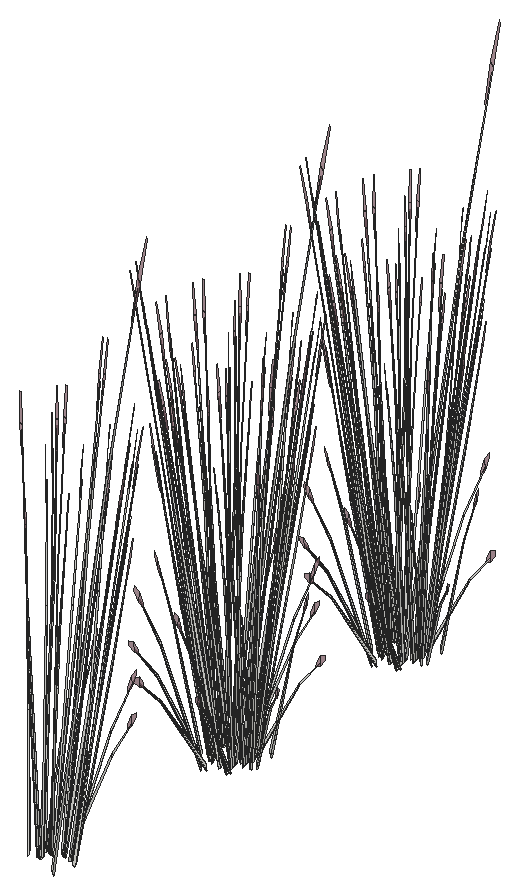
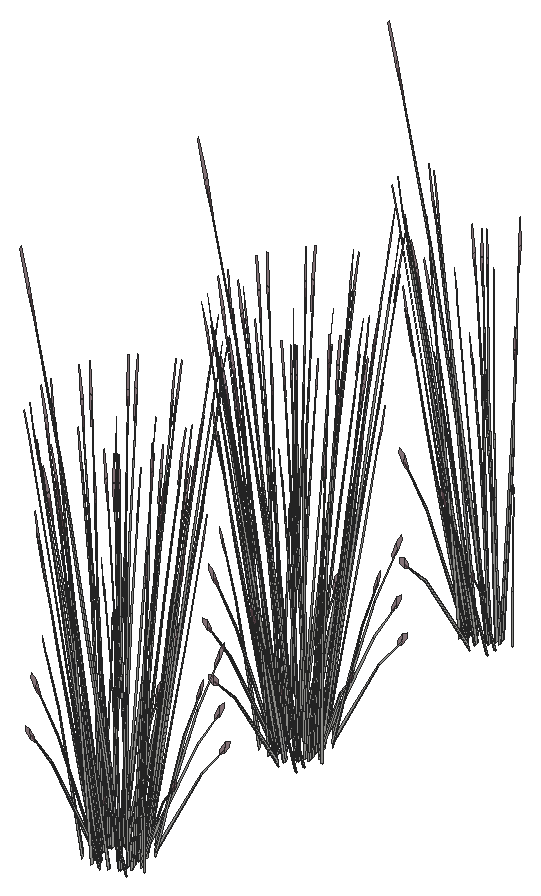
# SketchUp Ruby script. Lengths in inches.
U = 1.inch
M = Sketchup.active_model
def pt(a) = Geom::Point3d.new(a.map { |v| v * U })
def face(e, loops, mat)
  f = e.add_face(loops[0].map { |a| pt(a) })
  loops[1..].each { |l| e.add_face(l.map { |a| pt(a) }).erase! }
  f.material = f.back_material = mat if mat
  f
end
# faces: each face lists its corners as indices into pts; further lists are holes
def faces(e, pts, list, mat = nil) = list.each { |f| face(e, (f[0].is_a?(Array) ? f : [f]).map { |l| l.map { |i| pts[i] } }, mat) }
# xy, xz, yz: faces in a plane at the given z, y or x. An outline is a flat list of corners, or four numbers for a rectangle; further outlines are holes
def ring(l) = l.size == 4 ? [[l[0], l[1]], [l[2], l[1]], [l[2], l[3]], [l[0], l[3]]] : l.each_slice(2).to_a
def flat(e, list, mat, &to3) = list.each { |f| face(e, (f[0].is_a?(Array) ? f : [f]).map { |l| ring(l).map { |u, v| to3.(u, v) } }, mat) }
def xy(e, z, list, mat = nil) = flat(e, list, mat) { |x, y| [x, y, z] }
def xz(e, y, list, mat = nil) = flat(e, list, mat) { |x, z| [x, y, z] }
def yz(e, x, list, mat = nil) = flat(e, list, mat) { |y, z| [x, y, z] }
def lines(e, pts, list) = list.each { |a, b| e.add_line(pt(pts[a]), pt(pts[b])) }
# prism: a flat outline (further loops are holes) pulled along v
def prism(e, loops, v, mat = nil)
  f = face(e, loops, mat); d = Geom::Vector3d.new(v.map { |x| x * U })
  f.pushpull(f.normal.samedirection?(d) ? d.length : -d.length)
end
def box(e, o, s, mat = nil) = prism(e, [[o, [o[0] + s[0], o[1], o[2]], [o[0] + s[0], o[1] + s[1], o[2]], [o[0], o[1] + s[1], o[2]]]], [0, 0, s[2]], mat)
def at(x, y, z, deg = 0) = Geom::Transformation.translation(pt([x, y, z])) * Geom::Transformation.rotation(ORIGIN, Z_AXIS, deg.degrees)
def axes(o, x, y, z) = Geom::Transformation.new([*x, 0, *y, 0, *z, 0, *pt(o).to_a, 1])
def part(name) = M.definitions.add(name)
# library, detail: a bought-in or finely detailed component or shape, given as its bounding box
def library(name, o, s) = part(name).tap { |d| box(d.entities, o, s) }
def detail(e, o, s) = box(e.add_group.entities, o, s)
def put(e, d, t, mat = nil) = e.add_instance(d, t).tap { |i| i.material = mat if mat }
def group(e, t, mat = nil) = e.add_group.tap { |g| g.transformation = t; g.material = mat if mat }.entities
root = M.entities
M.materials.add("LightPink_Translucent").color = [144, 107, 117]
M.materials["LightPink_Translucent"].alpha = 0.75
c1 = part("blade")
p = [[2.15,0.21,22],[0,0.17,0],[0.09,0.45,0],[2.18,0.31,22],[2.29,0.31,22],[0.38,0.45,0],
  [2.48,0.24,33],[2.49,0.24,33],[2.48,0.22,33]]
faces(c1.entities,p,[[0,1,2,3],[4,5,2,3],[6,3,4,7],[8,0,3,6]])
c2 = part("seeds")
p = [[0.3,-0.1,1.38],[-0.01,-0.03,1.59],[-0.01,-0.03,0.03],[0.14,-0.07,-0.07],[0.29,-0.03,3],[0.15,0.01,3.11]]
faces(c2.entities,p,[[0,1,2,3],[1,0,4,5]],"LightPink_Translucent")
c3 = part("blade with seeds")
put(c3.entities,c1,at(0,0,0))
put(c3.entities,c2,axes([2.4,0.25,30.99],[1.5799,-0.05474,1.17369],[-0.12525,1.92788,0.29478],[-0.07173,-0.02425,1.56792]))
put(root,c3,axes([400.47,80.36,4.73],[-0.08753,-0.42921,0.48003],[0.34336,-0.07449,0.3958],[-0.1012,0.10094,0.9933]))
put(root,c3,axes([400.41,80.28,4.73],[-0.2423,-0.19613,0.0643],[0.14107,-0.2793,0.50621],[-0.07768,0.0903,0.77189]))
put(root,c3,axes([400.6875,80.22,5.05],[0.30722,-0.06665,0.35414],[0.08112,0.381,-0.4572],[-0.08804,0.10234,0.87481]))
put(root,c3,axes([399.5,80.05,4.71],[0.04504,0.01251,1.77383],[0.13934,0.41205,-0.16761],[-0.0922,0.10815,0.31391]))
put(root,c3,axes([403.32,81.08,4.73],[-0.01777,0.35463,0.0643],[-0.26836,-0.00972,0.50621],[0.1028,0.03711,0.77189]))
put(root,c3,axes([403.34,80.97,4.73],[-0.26024,0.30729,0.48003],[-0.22444,-0.32634,0.3958],[0.1221,0.05668,0.9933]))
put(root,c3,axes([399.99,81.3,5.65],[0.31145,0.12449,-0.06488],[-0.0958,0.38314,-0.29416],[-0.05094,0.05817,0.97024]))
put(root,c3,axes([402.52,81.32,5.05],[-0.05451,-0.37564,0.35414],[0.31161,-0.09919,-0.4572],[0.0837,0.10765,0.87481]))
put(root,c3,axes([402.72,79.16,4.47],[-0.30498,-0.24231,1.38283],[0.32203,-0.37727,0.59665],[0.0984,0.22736,1.33663]))
put(root,c3,axes([400.53,80.18,5.03],[0.32648,0.25715,-0.1216],[-0.18809,0.3724,-0.67495],[-0.09224,0.12945,1.02557]))
put(root,c3,axes([402.49,81.52,5.03],[0.21031,-0.39918,-0.1216],[0.30457,0.22997,-0.67495],[0.10587,0.11278,1.02557]))
put(root,c3,axes([401.1,80.98,5.05],[0.23881,-0.24554,0.35414],[0.22606,0.28036,-0.4572],[-0.0344,0.14245,0.87481]))
put(root,c3,axes([402.21,81.85,4.71],[0.00104,-0.05646,1.77383],[0.30246,-0.2491,-0.16761],[0.10506,0.08891,0.31391]))
put(root,c3,axes([400.88,81.2,4.73],[-0.29004,-0.02173,0.0643],[0.00795,-0.32812,0.50621],[-0.03035,0.12569,0.77189]))
put(root,c3,axes([400.98,81.23,4.73],[-0.25132,-0.3182,0.48003],[0.2669,-0.27442,0.3958],[-0.04636,0.14929,0.9933]))
put(root,c3,axes([401.77,81.38,5.05],[0.1064,-0.35863,0.35414],[0.31043,0.1046,-0.4572],[0.02846,0.14439,0.87481]))
put(root,c3,axes([402.56,81.66,4.73],[-0.16041,0.29625,0.0643],[-0.22843,-0.17248,0.50621],[0.07385,0.09498,0.77189]))
put(root,c3,axes([402.1875,82.66,5.65],[0.2439,-0.26754,-0.06488],[0.22348,0.29302,-0.29416],[0.01573,0.08303,0.97024]))
put(root,c3,axes([402.63,81.58,4.73],[-0.35104,0.10702,0.48003],[-0.06092,-0.41983,0.3958],[0.08256,0.12373,0.9933]))
put(root,c3,axes([401.67,81.71,4.73],[-0.26007,0.1585,0.0643],[-0.12729,-0.28902,0.50621],[0.02512,0.1274,0.77189]))
put(root,c3,axes([400.15,81.25,4.72],[-0.00877,0.09229,1.74944],[0.24897,0.32105,-0.27667],[-0.06518,0.15182,0.14031]))
put(root,c3,axes([400.95,81.05,5.4],[0.3879,0.02311,-0.13498],[-0.0106,0.43749,-0.74919],[-0.02694,0.1685,1.13838]))
put(root,c3,axes([401.67,81.53,5.03],[0.34538,-0.21713,-0.1216],[0.16972,0.38536,-0.67495],[0.04557,0.16239,1.02557]))
put(root,c3,axes([401.77,81.68,5.0625],[-0.34777,-0.12192,0.53283],[0.11892,-0.40083,0.43934],[0.0209,0.15763,1.10256]))
put(root,c3,axes([400.125,82.2,4.71],[0.04004,-0.02816,1.77383],[0.33095,0.18728,-0.16761],[-0.00778,0.15594,0.31391]))
put(root,c3,axes([401.58,82.4,4.72],[0.04474,0.0751,1.74944],[0.36104,0.0295,-0.27667],[0.03631,0.16562,0.14031]))
put(root,c3,axes([401.89,98.37,4.72],[-0.05398,-0.06539,1.74944],[-0.36026,0.04145,-0.27667],[-0.0575,-0.15639,0.14031]))
put(root,c3,axes([403.51,99.17,4.72],[-0.00341,-0.09282,1.74944],[-0.28775,-0.26825,-0.27667],[0.04449,-0.16261,0.14031]))
put(root,c3,axes([403.43,98.83,4.71],[-0.03584,0.03562,1.77383],[-0.35118,-0.12018,-0.16761],[-0.01271,-0.15545,0.31391]))
put(root,c3,axes([401.52,98.15,4.71],[-0.00658,0.0559,1.77383],[-0.32474,0.20287,-0.16761],[-0.09556,-0.1037,0.31391]))
put(root,c3,axes([401.45,99.14,5.09],[0.39316,-0.11987,0.53763],[0.06823,0.47021,0.4433],[-0.09247,-0.13858,1.11249]))
put(root,c3,axes([402.34,99.23,4.73],[0.34777,0.12192,0.48003],[-0.11892,0.40083,0.3958],[-0.0209,-0.15763,0.9933]))
put(root,c3,axes([402.4375,99.375,5.03],[-0.34538,0.21713,-0.1216],[-0.16972,-0.38536,-0.67495],[-0.04557,-0.16239,1.02557]))
put(root,c3,axes([403.15,99.86,5.03],[-0.3879,-0.02311,-0.1216],[0.0106,-0.43749,-0.67495],[0.02694,-0.1685,1.02557]))
put(root,c3,axes([402.43,99.2,4.73],[0.26007,-0.1585,0.0643],[0.12729,0.28902,0.50621],[-0.02512,-0.1274,0.77189]))
put(root,c3,axes([401.54,99.25,4.73],[0.16041,-0.29625,0.0643],[0.22843,0.17248,0.50621],[-0.07385,-0.09498,0.77189]))
put(root,c3,axes([402.33,99.53,5.05],[-0.1064,0.35863,0.35414],[-0.31043,-0.1046,-0.4572],[-0.02846,-0.14439,0.87481]))
put(root,c3,axes([403.125,99.68,4.73],[0.25132,0.3182,0.48003],[-0.2669,0.27442,0.3958],[0.04636,-0.14929,0.9933]))
put(root,c3,axes([401.61,99.21,5.43],[-0.23555,0.44708,-0.13619],[-0.34112,-0.25757,-0.75594],[-0.11858,-0.12631,1.14864]))
put(root,c3,axes([403.22,99.71,4.73],[0.29004,0.02173,0.0643],[-0.00795,0.32812,0.50621],[0.03035,-0.12569,0.77189]))
put(root,c3,axes([403,99.93,5.05],[-0.23881,0.24554,0.35414],[-0.22606,-0.28036,-0.4572],[0.0344,-0.14245,0.87481]))
put(root,c3,axes([400.71,99.09,4.72],[-0.07594,-0.00329,1.74944],[-0.24177,0.32918,-0.27667],[-0.129,-0.06726,0.14031]))
put(root,c3,axes([403.58,100.72,5.03],[-0.32648,-0.25715,-0.1216],[0.18809,-0.3724,-0.67495],[0.09224,-0.12945,1.02557]))
put(root,c3,axes([401.59,99.59,5.05],[0.05451,0.37564,0.35414],[-0.31161,0.09919,-0.4572],[-0.0837,-0.10765,0.87481]))
put(root,c3,axes([400.65,99.83,5.09],[0.29147,-0.34417,0.53763],[0.25138,0.3655,0.4433],[-0.13675,-0.06349,1.11249]))
put(root,c3,axes([404.38,100.61,4.71],[-0.0461,-0.00354,1.77383],[-0.19143,-0.37951,-0.16761],[0.07688,-0.12478,0.31391]))
put(root,c3,axes([400.78,99.83,4.73],[0.01777,-0.35463,0.0643],[0.26836,0.00972,0.50621],[-0.1028,-0.03711,0.77189]))
put(root,c3,axes([403.42,100.6875,5.05],[-0.30722,0.06665,0.35414],[-0.08112,-0.381,-0.4572],[0.08804,-0.10234,0.87481]))
put(root,c3,axes([403.7,100.63,4.73],[0.2423,0.19613,0.0643],[-0.14107,0.2793,0.50621],[0.07768,-0.0903,0.77189]))
put(root,c3,axes([403.63,100.55,4.73],[0.08753,0.42921,0.48003],[-0.34336,0.07449,0.3958],[0.1012,-0.10094,0.9933]))
put(root,c3,axes([404.55,101.07,4.72],[0.04898,-0.07104,1.74944],[-0.06269,-0.43574,-0.27667],[0.12289,-0.08262,0.14031]))
put(root,c3,axes([400.42,99.37,4.71],[0.02617,0.04654,1.77383],[-0.12614,0.41836,-0.16761],[-0.12775,0.00303,0.31391]))
put(root,c3,axes([400.97,100.09,5.05],[0.20082,0.29199,0.35414],[-0.2293,0.2764,-0.4572],[-0.1165,-0.04206,0.87481]))
put(root,c3,axes([400.91,99.91,5.03],[-0.0189,0.47427,-0.1216],[-0.35781,-0.01296,-0.67495],[-0.13781,-0.03295,1.02557]))
put(root,c3,axes([403.59,101.73,5.03],[-0.17758,-0.42229,-0.1216],[0.31518,-0.20752,-0.67495],[0.13282,-0.05572,1.02557]))
put(root,c3,axes([403.47,101.6,5.05],[-0.29332,-0.1301,0.35414],[0.08555,-0.37955,-0.4572],[0.11809,-0.0348,0.87481]))
put(root,c3,axes([400.4,100.91,4.73],[0.09971,-0.42522,0.48003],[0.32782,0.1454,0.3958],[-0.12892,0.02555,0.9933]))
put(root,c3,axes([400.37,100.79,4.73],[-0.12963,-0.31798,0.0643],[0.23638,-0.15564,0.50621],[-0.1042,0.03071,0.77189]))
put(root,c3,axes([403.73,101.72,4.73],[0.12963,0.31798,0.0643],[-0.23638,0.15564,0.50621],[0.1042,-0.03071,0.77189]))
put(root,c3,axes([403.71,101.61,4.73],[-0.09971,0.42522,0.48003],[-0.32782,-0.1454,0.3958],[0.12892,-0.02555,0.9933]))
put(root,c3,axes([400.64,100.91,5.05],[0.29332,0.1301,0.35414],[-0.08555,0.37955,-0.4572],[-0.11809,0.0348,0.87481]))
put(root,c3,axes([404.3,102.98,4.71],[-0.03191,-0.04083,1.77383],[0.06981,-0.43764,-0.16761],[0.12571,-0.02796,0.31391]))
put(root,c3,axes([400.14,101.21,4.72],[-0.05763,0.06055,1.74944],[0.0049,0.44239,-0.27667],[-0.13211,0.05753,0.14031]))
put(root,c3,axes([400.51,100.78,5.03],[0.17758,0.42229,-0.1216],[-0.31518,0.20752,-0.67495],[-0.13282,0.05572,1.02557]))
put(root,c3,axes([403.19,102.61,5.03],[0.0189,-0.47427,-0.1216],[0.35781,0.01296,-0.67495],[0.13781,0.03295,1.02557]))
put(root,c3,axes([403.14,102.42,5.05],[-0.20082,-0.29199,0.35414],[0.2293,-0.2764,-0.4572],[0.1165,0.04206,0.87481]))
put(root,c3,axes([403.5,102.32,4.72],[0.07571,-0.00789,1.74944],[0.20767,-0.36231,-0.27667],[0.13467,0.04783,0.14031]))
put(root,c3,axes([400.47,101.97,4.73],[-0.08753,-0.42921,0.48003],[0.34336,-0.07449,0.3958],[-0.1012,0.10094,0.9933]))
put(root,c3,axes([400.41,101.88,4.73],[-0.2423,-0.19613,0.0643],[0.14107,-0.2793,0.50621],[-0.07768,0.0903,0.77189]))
put(root,c3,axes([400.6875,101.82,5.05],[0.30722,-0.06665,0.35414],[0.08112,0.381,-0.4572],[-0.08804,0.10234,0.87481]))
put(root,c3,axes([399.5,101.65,4.71],[0.04504,0.01251,1.77383],[0.13934,0.41205,-0.16761],[-0.0922,0.10815,0.31391]))
put(root,c3,axes([403.32,102.68,4.73],[-0.01777,0.35463,0.0643],[-0.26836,-0.00972,0.50621],[0.1028,0.03711,0.77189]))
put(root,c3,axes([403.34,102.57,4.73],[-0.26024,0.30729,0.48003],[-0.22444,-0.32634,0.3958],[0.1221,0.05668,0.9933]))
put(root,c3,axes([399.99,102.9,5.65],[0.31145,0.12449,-0.06488],[-0.0958,0.38314,-0.29416],[-0.05094,0.05817,0.97024]))
put(root,c3,axes([402.52,102.93,5.05],[-0.05451,-0.37564,0.35414],[0.31161,-0.09919,-0.4572],[0.0837,0.10765,0.87481]))
put(root,c3,axes([402.72,100.77,4.47],[-0.30498,-0.24231,1.38283],[0.32203,-0.37727,0.59665],[0.0984,0.22736,1.33663]))
put(root,c3,axes([400.53,101.79,5.03],[0.32648,0.25715,-0.1216],[-0.18809,0.3724,-0.67495],[-0.09224,0.12945,1.02557]))
put(root,c3,axes([402.49,103.12,5.03],[0.21031,-0.39918,-0.1216],[0.30457,0.22997,-0.67495],[0.10587,0.11278,1.02557]))
put(root,c3,axes([401.1,102.58,5.05],[0.23881,-0.24554,0.35414],[0.22606,0.28036,-0.4572],[-0.0344,0.14245,0.87481]))
put(root,c3,axes([402.21,103.45,4.71],[0.00104,-0.05646,1.77383],[0.30246,-0.2491,-0.16761],[0.10506,0.08891,0.31391]))
put(root,c3,axes([400.88,102.8,4.73],[-0.29004,-0.02173,0.0643],[0.00795,-0.32812,0.50621],[-0.03035,0.12569,0.77189]))
put(root,c3,axes([400.98,102.83,4.73],[-0.25132,-0.3182,0.48003],[0.2669,-0.27442,0.3958],[-0.04636,0.14929,0.9933]))
put(root,c3,axes([401.77,102.99,5.05],[0.1064,-0.35863,0.35414],[0.31043,0.1046,-0.4572],[0.02846,0.14439,0.87481]))
put(root,c3,axes([402.56,103.27,4.73],[-0.16041,0.29625,0.0643],[-0.22843,-0.17248,0.50621],[0.07385,0.09498,0.77189]))
put(root,c3,axes([402.1875,104.27,5.65],[0.2439,-0.26754,-0.06488],[0.22348,0.29302,-0.29416],[0.01573,0.08303,0.97024]))
put(root,c3,axes([402.63,103.18,4.73],[-0.35104,0.10702,0.48003],[-0.06092,-0.41983,0.3958],[0.08256,0.12373,0.9933]))
put(root,c3,axes([401.67,103.3125,4.73],[-0.26007,0.1585,0.0643],[-0.12729,-0.28902,0.50621],[0.02512,0.1274,0.77189]))
put(root,c3,axes([400.15,102.86,4.72],[-0.00877,0.09229,1.74944],[0.24897,0.32105,-0.27667],[-0.06518,0.15182,0.14031]))
put(root,c3,axes([400.95,102.65,5.4],[0.3879,0.02311,-0.13498],[-0.0106,0.43749,-0.74919],[-0.02694,0.1685,1.13838]))
put(root,c3,axes([401.67,103.14,5.03],[0.34538,-0.21713,-0.1216],[0.16972,0.38536,-0.67495],[0.04557,0.16239,1.02557]))
put(root,c3,axes([401.77,103.28,5.0625],[-0.34777,-0.12192,0.53283],[0.11892,-0.40083,0.43934],[0.0209,0.15763,1.10256]))
put(root,c3,axes([400.125,103.8,4.71],[0.04004,-0.02816,1.77383],[0.33095,0.18728,-0.16761],[-0.00778,0.15594,0.31391]))
put(root,c3,axes([401.58,104,4.72],[0.04474,0.0751,1.74944],[0.36104,0.0295,-0.27667],[0.03631,0.16562,0.14031]))
put(root,c3,axes([401.89,118.46,4.72],[-0.05398,-0.06539,1.74944],[-0.36026,0.04145,-0.27667],[-0.0575,-0.15639,0.14031]))
put(root,c3,axes([403.51,119.26,4.72],[-0.00341,-0.09282,1.74944],[-0.28775,-0.26825,-0.27667],[0.04449,-0.16261,0.14031]))
put(root,c3,axes([403.43,118.93,4.71],[-0.03584,0.03562,1.77383],[-0.35118,-0.12018,-0.16761],[-0.01271,-0.15545,0.31391]))
put(root,c3,axes([401.52,118.24,4.71],[-0.00658,0.0559,1.77383],[-0.32474,0.20287,-0.16761],[-0.09556,-0.1037,0.31391]))
put(root,c3,axes([401.45,119.24,5.09],[0.39316,-0.11987,0.53763],[0.06823,0.47021,0.4433],[-0.09247,-0.13858,1.11249]))
put(root,c3,axes([402.34,119.32,4.73],[0.34777,0.12192,0.48003],[-0.11892,0.40083,0.3958],[-0.0209,-0.15763,0.9933]))
put(root,c3,axes([402.4375,119.47,5.03],[-0.34538,0.21713,-0.1216],[-0.16972,-0.38536,-0.67495],[-0.04557,-0.16239,1.02557]))
put(root,c3,axes([403.15,119.96,5.03],[-0.3879,-0.02311,-0.1216],[0.0106,-0.43749,-0.67495],[0.02694,-0.1685,1.02557]))
put(root,c3,axes([402.43,119.29,4.73],[0.26007,-0.1585,0.0643],[0.12729,0.28902,0.50621],[-0.02512,-0.1274,0.77189]))
put(root,c3,axes([401.54,119.34,4.73],[0.16041,-0.29625,0.0643],[0.22843,0.17248,0.50621],[-0.07385,-0.09498,0.77189]))
put(root,c3,axes([402.33,119.62,5.05],[-0.1064,0.35863,0.35414],[-0.31043,-0.1046,-0.4572],[-0.02846,-0.14439,0.87481]))
put(root,c3,axes([403.125,119.77,4.73],[0.25132,0.3182,0.48003],[-0.2669,0.27442,0.3958],[0.04636,-0.14929,0.9933]))
put(root,c3,axes([401.61,119.31,5.43],[-0.23555,0.44708,-0.13619],[-0.34112,-0.25757,-0.75594],[-0.11858,-0.12631,1.14864]))
put(root,c3,axes([403.22,119.8,4.73],[0.29004,0.02173,0.0643],[-0.00795,0.32812,0.50621],[0.03035,-0.12569,0.77189]))
put(root,c3,axes([403,120.02,5.05],[-0.23881,0.24554,0.35414],[-0.22606,-0.28036,-0.4572],[0.0344,-0.14245,0.87481]))
put(root,c3,axes([400.71,119.18,4.72],[-0.07594,-0.00329,1.74944],[-0.24177,0.32918,-0.27667],[-0.129,-0.06726,0.14031]))
put(root,c3,axes([403.58,120.82,5.03],[-0.32648,-0.25715,-0.1216],[0.18809,-0.3724,-0.67495],[0.09224,-0.12945,1.02557]))
put(root,c3,axes([401.59,119.68,5.05],[0.05451,0.37564,0.35414],[-0.31161,0.09919,-0.4572],[-0.0837,-0.10765,0.87481]))
put(root,c3,axes([400.65,119.92,5.09],[0.29147,-0.34417,0.53763],[0.25138,0.3655,0.4433],[-0.13675,-0.06349,1.11249]))
put(root,c3,axes([404.38,120.7,4.71],[-0.0461,-0.00354,1.77383],[-0.19143,-0.37951,-0.16761],[0.07688,-0.12478,0.31391]))
put(root,c3,axes([400.78,119.92,4.73],[0.01777,-0.35463,0.0643],[0.26836,0.00972,0.50621],[-0.1028,-0.03711,0.77189]))
put(root,c3,axes([403.42,120.78,5.05],[-0.30722,0.06665,0.35414],[-0.08112,-0.381,-0.4572],[0.08804,-0.10234,0.87481]))
put(root,c3,axes([403.7,120.72,4.73],[0.2423,0.19613,0.0643],[-0.14107,0.2793,0.50621],[0.07768,-0.0903,0.77189]))
put(root,c3,axes([403.63,120.64,4.73],[0.08753,0.42921,0.48003],[-0.34336,0.07449,0.3958],[0.1012,-0.10094,0.9933]))
put(root,c3,axes([404.55,121.16,4.72],[0.04898,-0.07104,1.74944],[-0.06269,-0.43574,-0.27667],[0.12289,-0.08262,0.14031]))
put(root,c3,axes([400.42,119.46,4.71],[0.02617,0.04654,1.77383],[-0.12614,0.41836,-0.16761],[-0.12775,0.00303,0.31391]))
put(root,c3,axes([400.97,120.19,5.05],[0.20082,0.29199,0.35414],[-0.2293,0.2764,-0.4572],[-0.1165,-0.04206,0.87481]))
put(root,c3,axes([400.91,120,5.03],[-0.0189,0.47427,-0.1216],[-0.35781,-0.01296,-0.67495],[-0.13781,-0.03295,1.02557]))
put(root,c3,axes([403.59,121.82,5.03],[-0.17758,-0.42229,-0.1216],[0.31518,-0.20752,-0.67495],[0.13282,-0.05572,1.02557]))
put(root,c3,axes([403.47,121.69,5.05],[-0.29332,-0.1301,0.35414],[0.08555,-0.37955,-0.4572],[0.11809,-0.0348,0.87481]))
put(root,c3,axes([400.4,121,4.73],[0.09971,-0.42522,0.48003],[0.32782,0.1454,0.3958],[-0.12892,0.02555,0.9933]))
put(root,c3,axes([400.37,120.89,4.73],[-0.12963,-0.31798,0.0643],[0.23638,-0.15564,0.50621],[-0.1042,0.03071,0.77189]))
put(root,c3,axes([403.73,121.81,4.73],[0.12963,0.31798,0.0643],[-0.23638,0.15564,0.50621],[0.1042,-0.03071,0.77189]))
put(root,c3,axes([403.71,121.7,4.73],[-0.09971,0.42522,0.48003],[-0.32782,-0.1454,0.3958],[0.12892,-0.02555,0.9933]))
put(root,c3,axes([400.64,121,5.05],[0.29332,0.1301,0.35414],[-0.08555,0.37955,-0.4572],[-0.11809,0.0348,0.87481]))
put(root,c3,axes([404.3,123.07,4.71],[-0.03191,-0.04083,1.77383],[0.06981,-0.43764,-0.16761],[0.12571,-0.02796,0.31391]))
put(root,c3,axes([400.14,121.3,4.72],[-0.05763,0.06055,1.74944],[0.0049,0.44239,-0.27667],[-0.13211,0.05753,0.14031]))
put(root,c3,axes([400.51,120.875,5.03],[0.17758,0.42229,-0.1216],[-0.31518,0.20752,-0.67495],[-0.13282,0.05572,1.02557]))
put(root,c3,axes([403.19,122.7,5.03],[0.0189,-0.47427,-0.1216],[0.35781,0.01296,-0.67495],[0.13781,0.03295,1.02557]))
put(root,c3,axes([403.14,122.51,5.05],[-0.20082,-0.29199,0.35414],[0.2293,-0.2764,-0.4572],[0.1165,0.04206,0.87481]))
put(root,c3,axes([403.5,122.41,4.72],[0.07571,-0.00789,1.74944],[0.20767,-0.36231,-0.27667],[0.13467,0.04783,0.14031]))
put(root,c3,axes([400.47,122.06,4.73],[-0.08753,-0.42921,0.48003],[0.34336,-0.07449,0.3958],[-0.1012,0.10094,0.9933]))
put(root,c3,axes([400.41,121.98,4.73],[-0.2423,-0.19613,0.0643],[0.14107,-0.2793,0.50621],[-0.07768,0.0903,0.77189]))
put(root,c3,axes([400.6875,121.92,5.05],[0.30722,-0.06665,0.35414],[0.08112,0.381,-0.4572],[-0.08804,0.10234,0.87481]))
put(root,c3,axes([399.5,121.75,4.71],[0.04504,0.01251,1.77383],[0.13934,0.41205,-0.16761],[-0.0922,0.10815,0.31391]))
put(root,c3,axes([403.32,122.78,4.73],[-0.01777,0.35463,0.0643],[-0.26836,-0.00972,0.50621],[0.1028,0.03711,0.77189]))
put(root,c3,axes([403.34,122.66,4.73],[-0.26024,0.30729,0.48003],[-0.22444,-0.32634,0.3958],[0.1221,0.05668,0.9933]))
put(root,c3,axes([399.99,123,5.65],[0.31145,0.12449,-0.06488],[-0.0958,0.38314,-0.29416],[-0.05094,0.05817,0.97024]))
put(root,c3,axes([402.52,123.02,5.05],[-0.05451,-0.37564,0.35414],[0.31161,-0.09919,-0.4572],[0.0837,0.10765,0.87481]))
put(root,c3,axes([402.72,120.86,4.47],[-0.30498,-0.24231,1.38283],[0.32203,-0.37727,0.59665],[0.0984,0.22736,1.33663]))
put(root,c3,axes([400.53,121.88,5.03],[0.32648,0.25715,-0.1216],[-0.18809,0.3724,-0.67495],[-0.09224,0.12945,1.02557]))
put(root,c3,axes([402.49,123.21,5.03],[0.21031,-0.39918,-0.1216],[0.30457,0.22997,-0.67495],[0.10587,0.11278,1.02557]))
put(root,c3,axes([401.1,122.67,5.05],[0.23881,-0.24554,0.35414],[0.22606,0.28036,-0.4572],[-0.0344,0.14245,0.87481]))
put(root,c3,axes([402.21,123.54,4.71],[0.00104,-0.05646,1.77383],[0.30246,-0.2491,-0.16761],[0.10506,0.08891,0.31391]))
put(root,c3,axes([400.88,122.9,4.73],[-0.29004,-0.02173,0.0643],[0.00795,-0.32812,0.50621],[-0.03035,0.12569,0.77189]))
put(root,c3,axes([400.98,122.93,4.73],[-0.25132,-0.3182,0.48003],[0.2669,-0.27442,0.3958],[-0.04636,0.14929,0.9933]))
put(root,c3,axes([401.77,123.08,5.05],[0.1064,-0.35863,0.35414],[0.31043,0.1046,-0.4572],[0.02846,0.14439,0.87481]))
put(root,c3,axes([402.56,123.36,4.73],[-0.16041,0.29625,0.0643],[-0.22843,-0.17248,0.50621],[0.07385,0.09498,0.77189]))
put(root,c3,axes([402.1875,124.36,5.65],[0.2439,-0.26754,-0.06488],[0.22348,0.29302,-0.29416],[0.01573,0.08303,0.97024]))
put(root,c3,axes([402.63,123.28,4.73],[-0.35104,0.10702,0.48003],[-0.06092,-0.41983,0.3958],[0.08256,0.12373,0.9933]))
put(root,c3,axes([401.67,123.4,4.73],[-0.26007,0.1585,0.0643],[-0.12729,-0.28902,0.50621],[0.02512,0.1274,0.77189]))
put(root,c3,axes([400.15,122.95,4.72],[-0.00877,0.09229,1.74944],[0.24897,0.32105,-0.27667],[-0.06518,0.15182,0.14031]))
